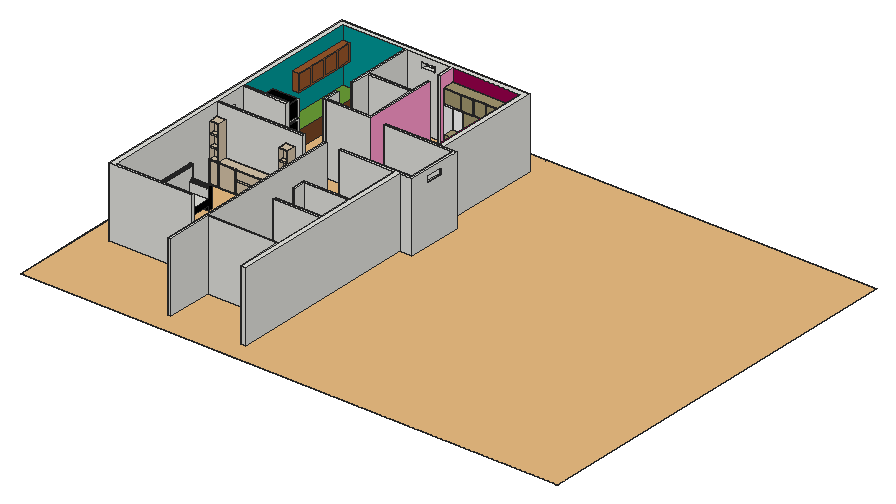
# SketchUp Ruby script. Lengths in millimetres.
U = 1.mm
M = Sketchup.active_model
def pt(a) = Geom::Point3d.new(a.map { |v| v * U })
def face(e, loops, mat)
  f = e.add_face(loops[0].map { |a| pt(a) })
  loops[1..].each { |l| e.add_face(l.map { |a| pt(a) }).erase! }
  f.material = f.back_material = mat if mat
  f
end
# faces: each face lists its corners as indices into pts; further lists are holes
def faces(e, pts, list, mat = nil) = list.each { |f| face(e, (f[0].is_a?(Array) ? f : [f]).map { |l| l.map { |i| pts[i] } }, mat) }
# xy, xz, yz: faces in a plane at the given z, y or x. An outline is a flat list of corners, or four numbers for a rectangle; further outlines are holes
def ring(l) = l.size == 4 ? [[l[0], l[1]], [l[2], l[1]], [l[2], l[3]], [l[0], l[3]]] : l.each_slice(2).to_a
def flat(e, list, mat, &to3) = list.each { |f| face(e, (f[0].is_a?(Array) ? f : [f]).map { |l| ring(l).map { |u, v| to3.(u, v) } }, mat) }
def xy(e, z, list, mat = nil) = flat(e, list, mat) { |x, y| [x, y, z] }
def xz(e, y, list, mat = nil) = flat(e, list, mat) { |x, z| [x, y, z] }
def yz(e, x, list, mat = nil) = flat(e, list, mat) { |y, z| [x, y, z] }
def lines(e, pts, list) = list.each { |a, b| e.add_line(pt(pts[a]), pt(pts[b])) }
# prism: a flat outline (further loops are holes) pulled along v
def prism(e, loops, v, mat = nil)
  f = face(e, loops, mat); d = Geom::Vector3d.new(v.map { |x| x * U })
  f.pushpull(f.normal.samedirection?(d) ? d.length : -d.length)
end
def box(e, o, s, mat = nil) = prism(e, [[o, [o[0] + s[0], o[1], o[2]], [o[0] + s[0], o[1] + s[1], o[2]], [o[0], o[1] + s[1], o[2]]]], [0, 0, s[2]], mat)
def at(x, y, z, deg = 0) = Geom::Transformation.translation(pt([x, y, z])) * Geom::Transformation.rotation(ORIGIN, Z_AXIS, deg.degrees)
def axes(o, x, y, z) = Geom::Transformation.new([*x, 0, *y, 0, *z, 0, *pt(o).to_a, 1])
def part(name) = M.definitions.add(name)
# library, detail: a bought-in or finely detailed component or shape, given as its bounding box
def library(name, o, s) = part(name).tap { |d| box(d.entities, o, s) }
def detail(e, o, s) = box(e.add_group.entities, o, s)
def put(e, d, t, mat = nil) = e.add_instance(d, t).tap { |i| i.material = mat if mat }
def group(e, t, mat = nil) = e.add_group.tap { |g| g.transformation = t; g.material = mat if mat }.entities
root = M.entities
M.materials.add("[Color H01]").color = [204, 255, 255]
M.materials.add("[Color H07]").color = [0, 153, 153]
M.materials.add("[Color L02]").color = [255, 153, 204]
M.materials.add("[Color L11]").color = [153, 0, 76]
M.materials.add("[Color M00]").color = [255, 255, 255]
M.materials.add("[Color M09]").color = [0, 0, 0]
M.materials.add("[Grass Dark Green]").color = [106, 157, 55]
M.materials.add("[Ornate Tile 02]").color = [201, 201, 201]
M.materials.add("[Tile Various Tan]").color = [214, 196, 169]
M.materials.add("[Wood Cherry Original]").color = [152, 86, 42]
M.materials.add("[Wood Lumber ButtJoined]").color = [164, 152, 112]
M.materials.add("[Wood Veneer 01]").color = [120, 70, 37]
c1 = library("DAY 6-A.dwg",[0,0,0],[23541.1,17455.5,0.1])
c2 = part("Component\#1")
xy(c2.entities,0,[[0,0,1144.4,1143]])
xy(c2.entities,1942.2,[[0,0,1144.4,40]])
xy(c2.entities,2054.6,[[0,0,1144.4,40]])
xy(c2.entities,3009.9,[[0,0,1144.4,1143]],"[Color M09]")
xz(c2.entities,0,[[[0,0,1144.4,1942.2],[23.7,24.4,1120.8,1917.8]],[[0,2054.6,1144.4,3009.9],[22.4,2077.6,1122.1,2986.9]]])
xz(c2.entities,0,[[23.7,24.4,1120.8,1917.8],[22.4,2077.6,1122.1,2986.9]],"[Color M09]")
xz(c2.entities,40,[[0,1942.2,1144.4,2054.6]],"[Color M09]")
xz(c2.entities,1143,[[0,0,1144.4,3009.9]],"[Color M09]")
yz(c2.entities,0,[[0,0,0,1942.2,40,1942.2,40,2054.6,0,2054.6,0,3009.9,1143,3009.9,1143,0]],"[Color M09]")
yz(c2.entities,1144.4,[[0,0,1143,0,1143,3009.9,0,3009.9,0,2054.6,40,2054.6,40,1942.2,0,1942.2]],"[Color M09]")
c3 = part("Single bed")
xy(c3.entities,0,[[0,0,1825,3282]])
xy(c3.entities,37.9,[[37.9,0,1787.1,38]],"[Wood Veneer 01]")
xy(c3.entities,85.7,[[0,85.7,53,3196.3],[1787,85.7,1825,3196.3]],"[Wood Veneer 01]")
xy(c3.entities,914.3,[[0,85.7,53,3196.3]])
xy(c3.entities,914.3,[[1787,85.7,1825,3196.3]],"[Wood Veneer 01]")
xy(c3.entities,962.1,[[37.9,0,1787.1,38]],"[Wood Veneer 01]")
xy(c3.entities,993.9,[[[122.3,122.3,1702.7,3153.7],[1037.3,2774.4,1637.3,3074.4],[237.3,2774.4,837.3,3074.4]]])
xy(c3.entities,993.9,[[146.1,3153.7,1678.9,3218.7]],"[Wood Veneer 01]")
xy(c3.entities,1000,[[0,0,1825,0,1825,3153.7,1702.7,3153.7,1702.7,122.3,122.3,122.3,122.3,3153.7,0,3153.7]],"[Wood Veneer 01]")
xy(c3.entities,1023.9,[[23.9,3153.7,146.1,3218.7],[1678.9,3153.7,1801.1,3218.7]],"[Wood Veneer 01]")
xy(c3.entities,1032.9,[[237.3,2774.4,837.3,3074.4],[1037.3,2774.4,1637.3,3074.4]])
xy(c3.entities,2018.1,[[23.9,3153.7,1801.1,3218.7]],"[Wood Veneer 01]")
xy(c3.entities,2042,[[0,3153.7,1825,3282]],"[Wood Veneer 01]")
xz(c3.entities,0,[[[0,0,1825,1000],[37.9,37.9,1787.1,962.1]]],"[Wood Veneer 01]")
xz(c3.entities,38,[[37.9,37.9,1787.1,962.1]],"[Wood Veneer 01]")
xz(c3.entities,85.7,[[0,85.7,53,914.3]])
xz(c3.entities,85.7,[[1787,85.7,1825,914.3]],"[Wood Veneer 01]")
xz(c3.entities,122.3,[[122.3,993.9,1702.7,1000]])
xz(c3.entities,2774.4,[[237.3,993.9,837.3,1032.9],[1037.3,993.9,1637.3,1032.9]])
xz(c3.entities,3074.4,[[237.3,993.9,837.3,1032.9],[1037.3,993.9,1637.3,1032.9]])
xz(c3.entities,3153.7,[[122.3,993.9,146.1,993.9,146.1,1023.9,23.9,1023.9,23.9,2018.1,1801.1,2018.1,1801.1,1023.9,1678.9,1023.9,1678.9,993.9,1702.7,993.9,1702.7,1000,1825,1000,1825,2042,0,2042,0,1000,122.3,1000]],"[Wood Veneer 01]")
xz(c3.entities,3196.3,[[0,85.7,53,914.3],[1787,85.7,1825,914.3]],"[Wood Veneer 01]")
xz(c3.entities,3218.7,[[146.1,993.9,1678.9,993.9,1678.9,1023.9,1801.1,1023.9,1801.1,2018.1,23.9,2018.1,23.9,1023.9,146.1,1023.9]])
xz(c3.entities,3282,[[0,0,1825,2042]],"[Wood Veneer 01]")
yz(c3.entities,0,[[[0,0,0,1000,3153.7,1000,3153.7,2042,3282,2042,3282,0],[85.7,85.7,3196.3,914.3]]],"[Wood Veneer 01]")
yz(c3.entities,23.9,[[3153.7,1023.9,3218.7,2018.1]],"[Wood Veneer 01]")
yz(c3.entities,37.9,[[0,37.9,38,962.1]],"[Wood Veneer 01]")
yz(c3.entities,53,[[85.7,85.7,3196.3,914.3]],"[Wood Veneer 01]")
yz(c3.entities,122.3,[[122.3,993.9,3153.7,1000]])
yz(c3.entities,146.1,[[3153.7,993.9,3218.7,1023.9]],"[Wood Veneer 01]")
yz(c3.entities,237.3,[[2774.4,993.9,3074.4,1032.9]])
yz(c3.entities,837.3,[[2774.4,993.9,3074.4,1032.9]])
yz(c3.entities,1037.3,[[2774.4,993.9,3074.4,1032.9]])
yz(c3.entities,1637.3,[[2774.4,993.9,3074.4,1032.9]])
yz(c3.entities,1678.9,[[3153.7,993.9,3218.7,1023.9]],"[Wood Veneer 01]")
yz(c3.entities,1702.7,[[122.3,993.9,3153.7,1000]])
yz(c3.entities,1787,[[85.7,85.7,3196.3,914.3]],"[Wood Veneer 01]")
yz(c3.entities,1787.1,[[0,37.9,38,962.1]],"[Wood Veneer 01]")
yz(c3.entities,1801.1,[[3153.7,1023.9,3218.7,2018.1]],"[Wood Veneer 01]")
yz(c3.entities,1825,[[[0,0,3282,0,3282,2042,3153.7,2042,3153.7,1000,0,1000],[85.7,85.7,3196.3,914.3]]],"[Wood Veneer 01]")
c4 = part("Component\#3")
xy(c4.entities,0,[[0,18,6874,2466]])
xy(c4.entities,99.3,[[99.3,0,6774.7,18]],"[Wood Veneer 01]")
xy(c4.entities,140.9,[[140.9,0,1757.8,18],[1840.9,0,5033.1,18],[5116.2,0,6733.1,18]],"[Wood Veneer 01]")
xy(c4.entities,1709.1,[[1840.9,0,5033.1,18]],"[Wood Veneer 01]")
xy(c4.entities,1792.2,[[1840.9,0,5033.1,18]],"[Wood Veneer 01]")
xy(c4.entities,3359.1,[[140.9,0,1757.8,18],[1840.9,0,5033.1,18],[5116.2,0,6733.1,18]],"[Wood Veneer 01]")
xy(c4.entities,3400.7,[[99.3,0,6774.7,18]],"[Wood Veneer 01]")
xy(c4.entities,3500,[[0,18,6874,2466]],"[Wood Veneer 01]")
xz(c4.entities,0,[[[99.3,99.3,6774.7,3400.7],[5116.2,140.9,6733.1,3359.1],[140.9,140.9,1757.8,3359.1],[1840.9,140.9,5033.1,1709.1],[1840.9,1792.2,5033.1,3359.1]]],"[Wood Veneer 01]")
xz(c4.entities,18,[[[0,0,6874,3500],[99.3,99.3,6774.7,3400.7]],[140.9,140.9,1757.8,3359.1],[1840.9,140.9,5033.1,1709.1],[5116.2,140.9,6733.1,3359.1],[1840.9,1792.2,5033.1,3359.1]],"[Wood Veneer 01]")
xz(c4.entities,2466,[[0,0,6874,3500]])
yz(c4.entities,0,[[18,0,2466,3500]],"[Wood Veneer 01]")
yz(c4.entities,99.3,[[0,99.3,18,3400.7]],"[Wood Veneer 01]")
yz(c4.entities,140.9,[[0,140.9,18,3359.1]],"[Wood Veneer 01]")
yz(c4.entities,1757.8,[[0,140.9,18,1750.7],[0,1750.7,18,3359.1]],"[Wood Veneer 01]")
yz(c4.entities,1840.9,[[0,140.9,18,1709.1],[0,1792.2,18,3359.1]],"[Wood Veneer 01]")
yz(c4.entities,5033.1,[[0,140.9,18,1709.1],[0,1792.2,18,3359.1]],"[Wood Veneer 01]")
yz(c4.entities,5116.2,[[0,140.9,18,1750.7],[0,1750.7,18,3359.1]],"[Wood Veneer 01]")
yz(c4.entities,6733.1,[[0,140.9,18,3359.1]],"[Wood Veneer 01]")
yz(c4.entities,6774.7,[[0,99.3,18,3400.7]],"[Wood Veneer 01]")
yz(c4.entities,6874,[[18,0,2466,3500]],"[Wood Veneer 01]")
c5 = part("High back sofa")
xy(c5.entities,0,[[0,0,0,1816,4458,1816,4458,1549,4457,1549,4457,0,4057,0,4057,1445,400,1445,400,0]],"[Color M09]")
xy(c5.entities,500,[[400,0,4057,1445]],"[Color M09]")
xy(c5.entities,1161,[[400,0,4057,1549]])
xy(c5.entities,2115,[[0,0,0.5,1549],[399.5,0,400,1549]])
xy(c5.entities,2150,[[4057,0,4057.5,1549],[4456.5,0,4457,1549]])
xz(c5.entities,0,[[4057,2131.5,4057,2138.2,4056.8,2132.6],[4057,2138.2,4057.5,2150,4057,2150]])
xz(c5.entities,0,[[0,0,400,0,400,500,4057,500,4057,0,4457,0,4457,2150,4456.5,2150,4457.2,2167.4,4445.9,2218.6,4421.7,2265.2,4386.3,2303.9,4342.1,2332.1,4292.1,2347.9,4257,2349.5,4239.6,2350.2,4188.4,2338.9,4141.8,2314.7,4103.1,2279.3,4074.9,2235.1,4059.1,2185.1,4057.5,2150,4057,2138.2,4057,1161,400,1161,400,2115,399.5,2115,392.7,2166.6,372.7,2214.7,341,2256,299.7,2287.7,251.6,2307.7,200,2314.5,148.4,2307.7,100.3,2287.7,59,2256,27.3,2214.7,7.3,2166.6,0.5,2115,0,2115]],"[Color M09]")
xz(c5.entities,1445,[[400,0,4057,500]],"[Color M09]")
xz(c5.entities,1549,[[4457,0,4458,0,4458,3496.2,4457,3496.2,4457,2168.5,4457.2,2167.4,4457,2161.8],[400,1161,4057,1161,4057,2150,4057.5,2150,4059.1,2185.1,4074.9,2235.1,4103.1,2279.3,4141.8,2314.7,4188.4,2338.9,4239.6,2350.2,4257,2349.5,4292.1,2347.9,4342.1,2332.1,4386.3,2303.9,4421.7,2265.2,4445.9,2218.6,4457,2168.5,4457,3496.2,0,3496.2,0,2115,0.5,2115,7.3,2166.6,27.3,2214.7,59,2256,100.3,2287.7,148.4,2307.7,200,2314.5,251.6,2307.7,299.7,2287.7,341,2256,372.7,2214.7,392.7,2166.6,399.5,2115,400,2115],[4456.5,2150,4457,2150,4457,2161.8]])
xz(c5.entities,1816,[[0,0,4458,3496.2]],"[Color M09]")
yz(c5.entities,0,[[0,0,0,2115,1549,2115,1549,3496.2,1548.5,3500,1553.1,3534.7,1566.5,3567,1587.7,3594.8,1615.5,3616,1647.8,3629.4,1682.5,3634,1717.2,3629.4,1749.5,3616,1777.3,3594.8,1798.5,3567,1811.9,3534.7,1816.5,3500,1816,3496.2,1816,0]],"[Color M09]")
yz(c5.entities,400,[[0,1161,1549,2115]])
yz(c5.entities,400,[[0,0,1445,500]],"[Color M09]")
yz(c5.entities,4057,[[0,1161,1549,2150]])
yz(c5.entities,4057,[[0,0,1445,500]],"[Color M09]")
yz(c5.entities,4457,[[0,0,1549,2150]],"[Color M09]")
yz(c5.entities,4458,[[1549,0,1816,0,1816,3496.2,1816.5,3500,1811.9,3534.7,1798.5,3567,1777.3,3594.8,1749.5,3616,1717.2,3629.4,1682.5,3634,1647.8,3629.4,1615.5,3616,1587.7,3594.8,1566.5,3567,1553.1,3534.7,1548.5,3500,1549,3496.2]],"[Color M09]")
p = [[0.5,0,2115],[7.3,0,2166.6],[7.3,1549,2166.6],[0.5,1549,2115],[392.7,0,2166.6],[399.5,0,2115],
  [399.5,1549,2115],[392.7,1549,2166.6],[4057.5,0,2150],[4059.1,0,2185.1],[4059.1,1549,2185.1],[4057.5,1549,2150],
  [4457.2,0,2167.4],[4456.5,0,2150],[4456.5,1549,2150],[4457,1549,2161.8],[4457.2,1549,2167.4],[27.3,0,2214.7],
  [27.3,1549,2214.7],[372.7,0,2214.7],[372.7,1549,2214.7],[4445.9,0,2218.6],[4457,1549,2168.5],[4445.9,1549,2218.6],
  [4074.9,0,2235.1],[4074.9,1549,2235.1],[59,0,2256],[59,1549,2256],[341,0,2256],[341,1549,2256],
  [4421.7,0,2265.2],[4421.7,1549,2265.2],[4103.1,0,2279.3],[4103.1,1549,2279.3],[100.3,0,2287.7],[100.3,1549,2287.7],
  [299.7,0,2287.7],[299.7,1549,2287.7],[4386.3,0,2303.9],[4386.3,1549,2303.9],[4141.8,0,2314.7],[4141.8,1549,2314.7],
  [148.4,0,2307.7],[148.4,1549,2307.7],[251.6,0,2307.7],[251.6,1549,2307.7],[4342.1,0,2332.1],[4342.1,1549,2332.1],
  [200,0,2314.5],[200,1549,2314.5],[4188.4,0,2338.9],[4188.4,1549,2338.9],[4292.1,0,2347.9],[4292.1,1549,2347.9],
  [4239.6,0,2350.2],[4239.6,1549,2350.2],[4257,0,2349.5],[4257,1549,2349.5],[4458,1549,3496.2],[4458,1548.5,3500],
  [4457,1548.5,3500],[0,1548.5,3500],[0,1549,3496.2],[4457,1549,3496.2],[4457,1816,3496.2],[0,1816,3496.2],
  [0,1816.5,3500],[4457,1816.5,3500],[4458,1816.5,3500],[4458,1816,3496.2],[4458,1553.1,3534.7],[4457,1553.1,3534.7],
  [0,1553.1,3534.7],[0,1811.9,3534.7],[4457,1811.9,3534.7],[4458,1811.9,3534.7],[4458,1566.5,3567],[4457,1566.5,3567],
  [0,1566.5,3567],[0,1798.5,3567],[4457,1798.5,3567],[4458,1798.5,3567],[4458,1587.7,3594.8],[4457,1587.7,3594.8],
  [0,1587.7,3594.8],[0,1777.3,3594.8],[4457,1777.3,3594.8],[4458,1777.3,3594.8],[4458,1615.5,3616],[4457,1615.5,3616],
  [0,1615.5,3616],[0,1749.5,3616],[4457,1749.5,3616],[4458,1749.5,3616],[4458,1647.8,3629.4],[4457,1647.8,3629.4],
  [0,1647.8,3629.4],[0,1717.2,3629.4],[4457,1717.2,3629.4],[4458,1717.2,3629.4],[4458,1682.5,3634],[4457,1682.5,3634],
  [0,1682.5,3634],[0,1549,3500],[4458,1816,3500],[4458,1549,3500],[0,1816,3500]]
faces(c5.entities,p,[[0,1,2,3],[4,5,6,7],[8,9,10,11],[12,13,14,15,16],[1,17,18,2],[19,4,7,20],[21,12,16,22,23],[9,24,25,10],
  [17,26,27,18],[28,19,20,29],[30,21,23,31],[24,32,33,25],[26,34,35,27],[36,28,29,37],[38,30,31,39],[32,40,41,33],
  [34,42,43,35],[44,36,37,45],[46,38,39,47],[42,48,49,43],[48,44,45,49],[40,50,51,41],[52,46,47,53],[50,54,55,51],
  [54,56,52,53,57,55],[58,59,60,61,62,63],[64,65,66,67,68,69],[59,70,71,72,61,60],[67,66,73,74,75,68],[70,76,77,78,72,71],[74,73,79,80,81,75],[76,82,83,84,78,77],
  [80,79,85,86,87,81],[82,88,89,90,84,83],[86,85,91,92,93,87],[88,94,95,96,90,89],[92,91,97,98,99,93],[94,100,101,102,96,95],[98,97,102,101,100,99]])
lines(c5.entities,p,[[62,103],[104,69],[58,105],[65,106]])
xy(root,0,[[5752.5,0,9144,914.4],[9144,0,10058.4,9330.7],[5752.5,914.4,5866.8,914.4,5866.8,2924.5,8915.4,2924.5,8915.4,914.4,9144,914.4,9144,9330.7,9699,9330.7,9699,11761.5,8915.4,11761.5,8915.4,11764.5,6613,11764.5,6613,11644.3,9582.5,11644.3,9582.5,9445,6484.9,9445,6484.9,9330.7,8915.4,9330.7,8915.4,6883.3,6895,6883.3,6895,6278.7,7009.3,6278.7,7009.3,6769,8915.4,6769,8915.4,5351.2,6895,5351.2,6895,5236.9,8915.4,5236.9,8915.4,2989.1,5866.8,2989.1,5866.8,9445,5752.5,9445],[5866.8,914.4,8915.4,2924.5],[0,3721,914.4,17373.6],
  [914.4,3721,4548.3,3721,4548.3,3835.3,1143,3835.3,1143,9330.7,4892.3,9330.7,4892.3,9445,1143,9445,1143,10735.8,3064,10735.8,3064,10850.1,1143,10850.1,1143,12376.4,1987.7,12376.4,1987.7,15654.3,3121.4,15654.3,3121.4,16230.6,3848.1,16230.6,3848.1,13280.6,3962.6,13280.6,3962.6,14054.7,3962.4,14054.7,3962.4,14164.8,3962.6,14164.8,3962.6,16230.6,5843.4,16230.6,5843.4,15559.9,5957.7,15559.9,5957.7,16230.6,8915.4,16230.6,8915.4,11764.5,9144,11764.5,9144,16459.2,914.4,16459.2],[9699,9330.7,10058.4,11761.5],[8915.4,11761.5,9144,11764.5],[9144,11761.5,9582.5,11764.5],[9699,11761.5,10058.4,11761.5,10058.4,17373.6,9144,17373.6,9144,11764.5,9699,11764.5],
  [9582.5,11761.5,9699,11764.5],[3962.4,14054.7,3962.6,14164.8],[5843.4,14054.7,5843.6,14164.8],[914.4,16459.2,9144,17373.6]])
xy(root,0,[[0,0,5752.5,3721]],"[Ornate Tile 02]")
xy(root,0,[[5866.8,2989.1,8915.4,2989.1,8915.4,5236.9,6895,5236.9,6895,5351.2,8915.4,5351.2,8915.4,6769,7009.3,6769,7009.3,6278.7,6895,6278.7,6895,6883.3,8915.4,6883.3,8915.4,9330.7,6484.9,9330.7,6484.9,9445,9582.5,9445,9582.5,11644.3,7124.1,11644.3,7124.1,10557.4,6616.1,10557.4,6616.1,11644.3,6613,11644.3,6613,11764.5,8915.4,11764.5,8915.4,15723.6,5957.7,15723.6,5957.7,15559.9,5843.4,15559.9,5843.4,16230.6,3962.6,16230.6,3962.6,14164.8,5843.4,14164.8,5843.4,14992.8,5957.7,14992.8,5957.7,11764.5,3962.6,11764.5,3962.6,11878.8,5843.4,11878.8,5843.4,14054.7,3962.6,14054.7,3962.6,13280.6,3848.1,13280.6,3848.1,15654.3,1987.7,15654.3,1987.7,12376.4,1143,12376.4,1143,10850.1,3064,10850.1,3064,10735.8,1143,10735.8,1143,9445,4892.3,9445,4892.3,9330.7,4562.1,9330.7,4562.1,8916.8,1143,8916.8,1143,3835.3,4548.3,3835.3,4548.3,3721,5752.5,3721,5752.5,9445,5866.8,9445]],"[Tile Various Tan]")
xy(root,9.4,[[5967,15723.6,6356.5,15730.6],[6416.5,15723.6,6806,15730.6],[6824.8,15723.6,7506,15730.6],[7524.8,15723.6,8206,15730.6],[8224.8,15723.6,8906,15730.6]],"[Color M00]")
xy(root,17.8,[[1160.8,8916.8,1526.2,8934.8],[1561.8,8916.8,2276.2,8934.8]],"[Tile Various Tan]")
xy(root,19.1,[[2313.1,8916.8,3393.9,8934.8]],"[Tile Various Tan]")
xy(root,20.3,[[3433.4,8916.8,4141.8,8934.8],[4183.4,8916.8,4541.8,8934.8]],"[Tile Various Tan]")
xy(root,27.4,[[3148.8,15654.3,3820.7,16280.3]],"[Wood Veneer 01]")
xy(root,300,[[2620.8,15881.8,2639.2,15884.2,2656.3,15891.3,2671,15902.6,2682.3,15917.3,2689.4,15934.4,2691.8,15952.8,2689.4,15971.2,2682.3,15988.3,2671,16003,2656.3,16014.3,2639.2,16021.4,2620.8,16023.8,2602.5,16021.4,2585.3,16014.3,2570.6,16003,2559.4,15988.3,2552.3,15971.2,2549.8,15952.8,2552.3,15934.4,2559.4,15917.3,2570.6,15902.6,2585.3,15891.3,2602.5,15884.2]])
xy(root,429.4,[[5967,15723.6,6356.5,15730.6],[6416.5,15723.6,6806,15730.6]],"[Color M00]")
xy(root,454.4,[[5967,15723.6,6806,15730.6]],"[Color M00]")
xy(root,475,[[[2293.1,15723.6,2968.9,16164.4],[2620.8,15881.8,2602.5,15884.2,2585.3,15891.3,2570.6,15902.6,2559.4,15917.3,2552.3,15934.4,2549.8,15952.8,2552.3,15971.2,2559.4,15988.3,2570.6,16003,2585.3,16014.3,2602.5,16021.4,2620.8,16023.8,2639.2,16021.4,2656.3,16014.3,2671,16003,2682.3,15988.3,2689.4,15971.2,2691.8,15952.8,2689.4,15934.4,2682.3,15917.3,2671,15902.6,2656.3,15891.3,2639.2,15884.2]]])
xy(root,530.9,[[2313.1,8916.8,3393.9,8934.8]],"[Tile Various Tan]")
xy(root,569.1,[[2313.1,8916.8,3393.9,8934.8]],"[Tile Various Tan]")
xy(root,663.5,[[5967,15730.6,6806,16168.6]],"[Wood Lumber ButtJoined]")
xy(root,672.6,[[3148.8,15654.3,3820.7,16280.3]])
xy(root,700,[[[1143,12376.4,1987.7,12376.4,1987.7,15654.3,3848.1,15654.3,3848.1,16230.6,1143,16230.6],[2267,15697.5,2995,16190.5]]],"[Grass Dark Green]")
xy(root,704,[[[2267,15697.5,2995,16190.5],[2293.1,15723.6,2968.9,16164.4]]])
xy(root,979.7,[[3433.4,8916.8,4141.8,8934.8],[4183.4,8916.8,4541.8,8934.8]],"[Tile Various Tan]")
xy(root,980.9,[[2313.1,8916.8,3393.9,8934.8]],"[Tile Various Tan]")
xy(root,982.2,[[1160.8,8916.8,1526.2,8934.8],[1561.8,8916.8,2276.2,8934.8]],"[Tile Various Tan]")
xy(root,1000,[[1143,8916.8,1543,8934.8],[1543,8916.8,4162.1,9330.7],[4162.1,8916.8,4562.1,8934.8]],"[Tile Various Tan]")
xy(root,1015.7,[[1158.7,8934.8,1527.3,9157.8],[4177.8,8934.8,4546.3,9157.8]],"[Tile Various Tan]")
xy(root,1484.3,[[1158.7,8934.8,1527.3,9157.8],[4177.8,8934.8,4546.3,9157.8]],"[Tile Various Tan]")
xy(root,1515.7,[[1158.7,8934.8,1527.3,9157.8],[4177.8,8934.8,4546.3,9157.8]],"[Tile Various Tan]")
xy(root,1718,[[1143,13430.6,1449,16230.6]])
xy(root,1741.7,[[1443,13454.3,1449,14106.9],[1443,14154.3,1449,14806.9],[1443,14854.3,1449,15506.9],[1443,15554.3,1449,16206.9]],"[Wood Cherry Original]")
xy(root,1840.6,[[5967,15723.6,6715.4,16168.6],[6715.4,15723.6,6806,16168.6],[6824.8,15723.6,7265.4,15730.6],[7265.4,15723.6,7506,15730.6],[7524.8,15723.6,7815.4,15730.6],
  [7815.4,15723.6,8206,15730.6],[8224.8,15723.6,8365.4,15730.6],[8365.4,15723.6,8906,15730.6]],"[Color M00]")
xy(root,1859.4,[[5967,15723.6,6706,15730.6],[6724.8,15723.6,6815.4,15730.6],[6815.4,15723.6,7256,15730.6],[7274.8,15723.6,7515.4,15730.6],[7515.4,15723.6,7806,15730.6],
  [7824.8,15723.6,8215.4,15730.6],[8215.4,15723.6,8356,15730.6],[8374.8,15723.6,8906,15730.6]],"[Color M00]")
xy(root,1984.3,[[1158.7,8934.8,1527.3,9157.8],[4177.8,8934.8,4546.3,9157.8]],"[Tile Various Tan]")
xy(root,2015.7,[[1158.7,8934.8,1527.3,9157.8],[4177.8,8934.8,4546.3,9157.8]],"[Tile Various Tan]")
xy(root,2332.1,[[914.4,9911,1143,10360]])
xy(root,2444.3,[[1443,13454.3,1449,14106.9],[1443,14154.3,1449,14806.9],[1443,14854.3,1449,15506.9],[1443,15554.3,1449,16206.9]],"[Wood Cherry Original]")
xy(root,2466.9,[[9582.5,10139.4,9699,10982.4]])
xy(root,2468,[[1143,13430.6,1449,16230.6]],"[Wood Cherry Original]")
xy(root,2484.3,[[1158.7,8934.8,1527.3,9157.8],[4177.8,8934.8,4546.3,9157.8]],"[Tile Various Tan]")
xy(root,2490.6,[[5967,15723.6,6706,15730.6],[6724.8,15723.6,7256,15730.6],[7274.8,15723.6,7806,15730.6],[7824.8,15723.6,8356,15730.6],[8374.8,15723.6,8906,15730.6]],"[Color M00]")
xy(root,2500,[[1143,8934.8,1543,9330.7],[4162.1,8934.8,4562.1,9330.7]],"[Tile Various Tan]")
xy(root,2500,[[5957.7,15723.6,8915.4,16230.6]],"[Wood Lumber ButtJoined]")
xy(root,2571.4,[[4607.3,16230.6,5189.3,16459.2]])
xy(root,2576.1,[[914.4,9911,1143,10360]])
xy(root,2784.9,[[9582.5,10139.4,9699,10982.4]])
xy(root,2828.4,[[4607.3,16230.6,5189.3,16459.2]])
xy(root,3048,[[5752.5,914.4,5866.8,914.4,5866.8,2924.5,8915.4,2924.5,8915.4,914.4,9144,914.4,9144,9330.7,9699,9330.7,9699,11761.5,8915.4,11761.5,8915.4,11764.5,6613,11764.5,6613,11644.3,9582.5,11644.3,9582.5,9445,6484.9,9445,6484.9,9330.7,8915.4,9330.7,8915.4,6883.3,6895,6883.3,6895,6278.7,7009.3,6278.7,7009.3,6769,8915.4,6769,8915.4,5351.2,6895,5351.2,6895,5236.9,8915.4,5236.9,8915.4,2989.1,5866.8,2989.1,5866.8,9445,5752.5,9445],[914.4,3721,4548.3,3721,4548.3,3835.3,1143,3835.3,1143,9330.7,4892.3,9330.7,4892.3,9445,1143,9445,1143,10735.8,3064,10735.8,3064,10850.1,1143,10850.1,1143,16230.6,3848.1,16230.6,3848.1,13280.6,3962.6,13280.6,3962.6,14054.7,3962.4,14054.7,3962.4,14164.8,3962.6,14164.8,3962.6,16230.6,5843.4,16230.6,5843.4,15559.9,5957.7,15559.9,5957.7,16230.6,8915.4,16230.6,8915.4,11764.5,9144,11764.5,9144,16459.2,914.4,16459.2],[3848.1,11764.5,3962.4,12495.9],[3962.6,11764.5,5957.7,11764.5,5957.7,14992.8,5843.4,14992.8,5843.4,14164.8,5843.6,14164.8,5843.6,14054.7,5843.4,14054.7,5843.4,11878.8,3962.6,11878.8],[3962.6,14054.7,5843.4,14164.8]])
xz(root,914.4,[[5752.5,0,5866.8,3048],[8915.4,0,9144,3048]])
xz(root,2924.5,[[5866.8,0,8915.4,3048]])
xz(root,2989.1,[[5866.8,0,8915.4,3048]])
xz(root,3721,[[914.4,0,4548.3,3048]])
xz(root,3835.3,[[1143,0,4548.3,3048]])
xz(root,5236.9,[[6895,0,8915.4,3048]])
xz(root,5351.2,[[6895,0,8915.4,3048]])
xz(root,6278.7,[[6895,0,7009.3,3048]])
xz(root,6769,[[7009.3,0,8915.4,3048]])
xz(root,6883.3,[[6895,0,7009.3,3048],[7009.3,0,8915.4,3048]])
xz(root,8916.8,[[[1143,0,4562.1,1000],[1561.8,17.8,2276.2,982.2],[3433.4,20.3,4141.8,979.7],[2313.1,19.1,3393.9,530.9],[2313.1,569.1,3393.9,980.9],[1160.8,17.8,1526.2,982.2],[4183.4,20.3,4541.8,979.7]]],"[Tile Various Tan]")
xz(root,8934.8,[[1160.8,17.8,1526.2,982.2],[1561.8,17.8,2276.2,982.2],[2313.1,19.1,3393.9,530.9],[3433.4,20.3,4141.8,979.7],[4183.4,20.3,4541.8,979.7],
  [2313.1,569.1,3393.9,980.9],[[1143,1000,1543,2500],[1158.7,2015.7,1527.3,2484.3],[1158.7,1515.7,1527.3,1984.3],[1158.7,1015.7,1527.3,1484.3]],[[4162.1,1000,4562.1,2500],[4177.8,2015.7,4546.3,2484.3],[4177.8,1515.7,4546.3,1984.3],[4177.8,1015.7,4546.3,1484.3]]],"[Tile Various Tan]")
xz(root,9157.8,[[1158.7,1015.7,1527.3,1484.3],[4177.8,1015.7,4546.3,1484.3],[1158.7,1515.7,1527.3,1984.3],[4177.8,1515.7,4546.3,1984.3],[1158.7,2015.7,1527.3,2484.3],
  [4177.8,2015.7,4546.3,2484.3]],"[Tile Various Tan]")
xz(root,9330.7,[[4562.1,0,4892.3,0,4892.3,3048,1143,3048,1143,2500,1543,2500,1543,1000,4162.1,1000,4162.1,2500,4562.1,2500],[6484.9,0,8915.4,3048],[9144,0,9699,3048]])
xz(root,9330.7,[[1143,0,4562.1,0,4562.1,2500,4162.1,2500,4162.1,1000,1543,1000,1543,2500,1143,2500]],"[Tile Various Tan]")
xz(root,9445,[[1143,0,4892.3,3048],[5752.5,0,5866.8,3048],[6484.9,0,9582.5,3048]])
xz(root,9911,[[914.4,2332.1,1143,2576.1]])
xz(root,10139.4,[[9582.5,2466.9,9699,2784.9]])
xz(root,10360,[[914.4,2332.1,1143,2576.1]])
xz(root,10735.8,[[1143,0,3064,3048]])
xz(root,10850.1,[[1143,0,3064,3048]],"[Color H07]")
xz(root,10982.4,[[9582.5,2466.9,9699,2784.9]])
xz(root,11644.3,[[6613,0,6616.1,3048],[6616.1,0,9582.5,3048]])
xz(root,11761.5,[[8915.4,0,9144,3048],[9144,0,9699,3048]])
xz(root,11764.5,[[3848.1,0,3962.4,3048],[3962.6,0,5957.7,3048],[8915.4,0,9144,3048]])
xz(root,11764.5,[[6613,0,8915.4,3048]],"[Color L11]")
xz(root,11878.8,[[3962.6,0,5843.4,3048]])
xz(root,12376.4,[[1143,0,1987.7,700]])
xz(root,12495.9,[[3848.1,0,3962.4,3048]])
xz(root,13280.6,[[3848.1,0,3962.6,3048]])
xz(root,13430.6,[[1143,1718,1449,2468]],"[Wood Cherry Original]")
xz(root,13454.3,[[1443,1741.7,1449,2444.3]],"[Wood Cherry Original]")
xz(root,14054.7,[[3962.4,0,3962.6,3048],[3962.6,0,5843.4,3048],[5843.4,0,5843.6,3048]])
xz(root,14106.9,[[1443,1741.7,1449,2444.3]],"[Wood Cherry Original]")
xz(root,14154.3,[[1443,1741.7,1449,2444.3]],"[Wood Cherry Original]")
xz(root,14164.8,[[3962.4,0,3962.6,3048],[3962.6,0,5843.4,3048],[5843.4,0,5843.6,3048]])
xz(root,14806.9,[[1443,1741.7,1449,2444.3]],"[Wood Cherry Original]")
xz(root,14854.3,[[1443,1741.7,1449,2444.3]],"[Wood Cherry Original]")
xz(root,14992.8,[[5843.4,0,5957.7,3048]])
xz(root,15506.9,[[1443,1741.7,1449,2444.3]],"[Wood Cherry Original]")
xz(root,15554.3,[[1443,1741.7,1449,2444.3]],"[Wood Cherry Original]")
xz(root,15559.9,[[5843.4,0,5957.7,3048]])
xz(root,15654.3,[[[1987.7,0,3848.1,700],[3148.8,27.4,3820.7,672.6]]],"[Wood Veneer 01]")
xz(root,15697.5,[[2267,700,2995,704]])
xz(root,15723.6,[[2293.1,475,2968.9,704]])
xz(root,15723.6,[[[5957.7,0,8915.4,2500],[5967,9.4,6806,1840.6],[8224.8,9.4,8906,1840.6],[6824.8,9.4,7506,1840.6],[7524.8,9.4,8206,1840.6],[5967,1859.4,6706,2490.6],[6724.8,1859.4,7256,2490.6],[7274.8,1859.4,7806,2490.6],[8374.8,1859.4,8906,2490.6],[7824.8,1859.4,8356,2490.6]],[6356.5,9.4,6416.5,9.4,6416.5,429.4,6806,429.4,6806,454.4,5967,454.4,5967,429.4,6356.5,429.4]],"[Color M00]")
xz(root,15730.6,[[5967,9.4,6356.5,429.4],[6416.5,9.4,6806,429.4],[6824.8,9.4,7506,1840.6],[7524.8,9.4,8206,1840.6],[8224.8,9.4,8906,1840.6],
  [5967,454.4,6806,663.5],[5967,1859.4,6706,2490.6],[6724.8,1859.4,7256,2490.6],[7274.8,1859.4,7806,2490.6],[7824.8,1859.4,8356,2490.6],
  [8374.8,1859.4,8906,2490.6]],"[Wood Lumber ButtJoined]")
xz(root,16164.4,[[2293.1,475,2968.9,704]])
xz(root,16190.5,[[2267,700,2995,704]])
xz(root,16206.9,[[1443,1741.7,1449,2444.3]],"[Wood Cherry Original]")
xz(root,16230.6,[[3121.4,0,3848.1,700],[[3962.6,0,5843.4,3048],[4607.3,2571.4,5189.3,2828.4]]])
xz(root,16230.6,[[1143,700,3848.1,700,3848.1,3048,1143,3048,1143,2468,1449,2468,1449,1718,1143,1718]],"[Color H07]")
xz(root,16230.6,[[5957.7,2500,8915.4,3048]],"[Color L11]")
xz(root,16230.6,[[5957.7,0,8915.4,2500]],"[Color M00]")
xz(root,16280.3,[[3148.8,27.4,3820.7,672.6]])
xz(root,16459.2,[[[914.4,0,9144,3048],[4607.3,2571.4,5189.3,2828.4]]])
yz(root,914.4,[[[3721,0,16459.2,3048],[9911,2332.1,10360,2576.1]]])
yz(root,1143,[[3835.3,0,8916.8,0,8916.8,1000,8934.8,1000,8934.8,2500,9330.7,2500,9330.7,3048,3835.3,3048],[[9445,0,10735.8,3048],[9911,2332.1,10360,2576.1]]])
yz(root,1143,[[10850.1,0,12376.4,0,12376.4,700,16230.6,700,16230.6,1718,13430.6,1718,13430.6,2468,16230.6,2468,16230.6,3048,10850.1,3048]],"[Color H07]")
yz(root,1143,[[8916.8,0,9330.7,0,9330.7,2500,8934.8,2500,8934.8,1000,8916.8,1000]],"[Tile Various Tan]")
yz(root,1158.7,[[8934.8,1015.7,9157.8,1484.3],[8934.8,1515.7,9157.8,1984.3],[8934.8,2015.7,9157.8,2484.3]],"[Tile Various Tan]")
yz(root,1160.8,[[8916.8,17.8,8934.8,982.2]],"[Tile Various Tan]")
yz(root,1443,[[13454.3,1741.7,14106.9,2444.3],[14154.3,1741.7,14806.9,2444.3],[14854.3,1741.7,15506.9,2444.3],[15554.3,1741.7,16206.9,2444.3]],"[Wood Cherry Original]")
yz(root,1449,[[[13430.6,1718,16230.6,2468],[14854.3,1741.7,15506.9,2444.3],[13454.3,1741.7,14106.9,2444.3],[15554.3,1741.7,16206.9,2444.3],[14154.3,1741.7,14806.9,2444.3]]],"[Wood Cherry Original]")
yz(root,1526.2,[[8916.8,17.8,8934.8,982.2]],"[Tile Various Tan]")
yz(root,1527.3,[[8934.8,1015.7,9157.8,1484.3],[8934.8,1515.7,9157.8,1984.3],[8934.8,2015.7,9157.8,2484.3]],"[Tile Various Tan]")
yz(root,1543,[[8934.8,1000,9330.7,2500]],"[Tile Various Tan]")
yz(root,1561.8,[[8916.8,17.8,8934.8,982.2]],"[Tile Various Tan]")
yz(root,1987.7,[[12376.4,0,15654.3,700]],"[Wood Veneer 01]")
yz(root,2267,[[15697.5,700,16190.5,704]])
yz(root,2276.2,[[8916.8,17.8,8934.8,550],[8916.8,550,8934.8,982.2]],"[Tile Various Tan]")
yz(root,2293.1,[[15723.6,475,16164.4,704]])
yz(root,2313.1,[[8916.8,19.1,8934.8,530.9],[8916.8,569.1,8934.8,980.9]],"[Tile Various Tan]")
yz(root,2968.9,[[15723.6,475,16164.4,704]])
yz(root,2995,[[15697.5,700,16190.5,704]])
yz(root,3064,[[10735.8,0,10850.1,3048]])
yz(root,3148.8,[[15654.3,27.4,16280.3,672.6]],"[Wood Veneer 01]")
yz(root,3393.9,[[8916.8,19.1,8934.8,530.9],[8916.8,569.1,8934.8,980.9]],"[Tile Various Tan]")
yz(root,3433.4,[[8916.8,20.3,8934.8,550],[8916.8,550,8934.8,979.7]],"[Tile Various Tan]")
yz(root,3820.7,[[15654.3,27.4,16280.3,672.6]],"[Wood Veneer 01]")
yz(root,3848.1,[[15654.3,0,16230.6,700]])
yz(root,3848.1,[[11764.5,0,12495.9,3048],[13280.6,0,13280.6,3048,16230.6,3048,16230.6,700,15654.3,700,15654.3,0]],"[Color H01]")
yz(root,3962.4,[[11764.5,0,12495.9,3048],[14054.7,0,14164.8,3048]])
yz(root,3962.6,[[11764.5,0,11878.8,3048],[13280.6,0,14054.7,3048],[14054.7,0,14164.8,3048],[14164.8,0,16230.6,3048]])
yz(root,4141.8,[[8916.8,20.3,8934.8,979.7]],"[Tile Various Tan]")
yz(root,4162.1,[[8934.8,1000,9330.7,2500]],"[Tile Various Tan]")
yz(root,4177.8,[[8934.8,1015.7,9157.8,1484.3],[8934.8,1515.7,9157.8,1984.3],[8934.8,2015.7,9157.8,2484.3]],"[Tile Various Tan]")
yz(root,4183.4,[[8916.8,20.3,8934.8,979.7]],"[Tile Various Tan]")
yz(root,4541.8,[[8916.8,20.3,8934.8,979.7]],"[Tile Various Tan]")
yz(root,4546.3,[[8934.8,1015.7,9157.8,1484.3],[8934.8,1515.7,9157.8,1984.3],[8934.8,2015.7,9157.8,2484.3]],"[Tile Various Tan]")
yz(root,4548.3,[[3721,0,3835.3,3048]])
yz(root,4562.1,[[8916.8,0,9330.7,0,9330.7,2500,8934.8,2500,8934.8,1000,8916.8,1000]],"[Tile Various Tan]")
yz(root,4607.3,[[16230.6,2571.4,16459.2,2828.4]])
yz(root,4892.3,[[9330.7,0,9445,3048]])
yz(root,5189.3,[[16230.6,2571.4,16459.2,2828.4]])
yz(root,5752.5,[[914.4,0,9445,3048]])
yz(root,5843.4,[[11878.8,0,14054.7,3048],[14054.7,0,14164.8,3048],[14164.8,0,14992.8,3048],[15559.9,0,16230.6,3048]])
yz(root,5843.6,[[14054.7,0,14164.8,3048]])
yz(root,5866.8,[[914.4,0,2924.5,3048],[2989.1,0,9445,3048]])
yz(root,5957.7,[[11764.5,0,14992.8,3048],[15559.9,0,15723.6,0,15723.6,2500,16230.6,2500,16230.6,3048,15559.9,3048]],"[Color L02]")
yz(root,5957.7,[[15723.6,0,16230.6,2500]],"[Color M00]")
yz(root,5967,[[15723.6,9.4,15730.6,429.4],[15723.6,454.4,15730.6,454.4,15730.6,663.5,16168.6,663.5,16168.6,1840.6,15723.6,1840.6],[15723.6,1859.4,15730.6,2490.6]],"[Color M00]")
yz(root,6356.5,[[15723.6,9.4,15730.6,429.4]],"[Color M00]")
yz(root,6416.5,[[15723.6,9.4,15730.6,429.4]],"[Color M00]")
yz(root,6484.9,[[9330.7,0,9445,3048]])
yz(root,6613,[[11644.3,0,11764.5,3048]])
yz(root,6706,[[15723.6,1859.4,15730.6,2490.6]],"[Color M00]")
yz(root,6724.8,[[15723.6,1859.4,15730.6,2490.6]],"[Color M00]")
yz(root,6806,[[15723.6,9.4,15730.6,429.4],[15723.6,454.4,15723.6,1840.6,16168.6,1840.6,16168.6,663.5,15730.6,663.5,15730.6,454.4]],"[Color M00]")
yz(root,6824.8,[[15723.6,9.4,15730.6,1840.6]],"[Color M00]")
yz(root,6895,[[5236.9,0,5351.2,3048],[6278.7,0,6883.3,3048]])
yz(root,7009.3,[[6278.7,0,6769,3048]])
yz(root,7256,[[15723.6,1859.4,15730.6,2490.6]],"[Color M00]")
yz(root,7274.8,[[15723.6,1859.4,15730.6,2490.6]],"[Color M00]")
yz(root,7506,[[15723.6,9.4,15730.6,1840.6]],"[Color M00]")
yz(root,7524.8,[[15723.6,9.4,15730.6,1840.6]],"[Color M00]")
yz(root,7806,[[15723.6,1859.4,15730.6,2490.6]],"[Color M00]")
yz(root,7824.8,[[15723.6,1859.4,15730.6,2490.6]],"[Color M00]")
yz(root,8206,[[15723.6,9.4,15730.6,1840.6]],"[Color M00]")
yz(root,8224.8,[[15723.6,9.4,15730.6,1840.6]],"[Color M00]")
yz(root,8356,[[15723.6,1859.4,15730.6,2490.6]],"[Color M00]")
yz(root,8374.8,[[15723.6,1859.4,15730.6,2490.6]],"[Color M00]")
yz(root,8906,[[15723.6,9.4,15730.6,1840.6],[15723.6,1859.4,15730.6,2490.6]],"[Color M00]")
yz(root,8915.4,[[914.4,0,2924.5,3048],[2989.1,0,5236.9,3048],[5351.2,0,6769,3048],[6883.3,0,9330.7,3048],[11761.5,0,11764.5,3048]])
yz(root,8915.4,[[11764.5,0,11764.5,3048,16230.6,3048,16230.6,2500,15723.6,2500,15723.6,0]],"[Color L11]")
yz(root,8915.4,[[15723.6,0,16230.6,2500]],"[Tile Various Tan]")
yz(root,9144,[[914.4,0,9330.7,3048],[11764.5,0,16459.2,3048]])
yz(root,9582.5,[[[9445,0,11644.3,3048],[10139.4,2466.9,10982.4,2784.9]]])
yz(root,9699,[[[9330.7,0,11761.5,3048],[10139.4,2466.9,10982.4,2784.9]]])
p = [[2602.5,15884.2,475],[2620.8,15881.8,475],[2620.8,15881.8,300],[2602.5,15884.2,300],[2639.2,15884.2,475],[2639.2,15884.2,300],
  [2585.3,15891.3,475],[2585.3,15891.3,300],[2656.3,15891.3,475],[2656.3,15891.3,300],[2570.6,15902.6,475],[2570.6,15902.6,300],
  [2671,15902.6,475],[2671,15902.6,300],[2559.4,15917.3,475],[2559.4,15917.3,300],[2682.3,15917.3,475],[2682.3,15917.3,300],
  [2552.3,15934.4,475],[2552.3,15934.4,300],[2689.4,15934.4,475],[2689.4,15934.4,300],[2549.8,15952.8,475],[2549.8,15952.8,300],
  [2691.8,15952.8,475],[2691.8,15952.8,300],[2552.3,15971.2,475],[2552.3,15971.2,300],[2689.4,15971.2,475],[2689.4,15971.2,300],
  [2559.4,15988.3,475],[2559.4,15988.3,300],[2682.3,15988.3,475],[2682.3,15988.3,300],[2570.6,16003,475],[2570.6,16003,300],
  [2671,16003,475],[2671,16003,300],[2585.3,16014.3,475],[2585.3,16014.3,300],[2656.3,16014.3,475],[2656.3,16014.3,300],
  [2602.5,16021.4,475],[2602.5,16021.4,300],[2639.2,16021.4,475],[2639.2,16021.4,300],[2620.8,16023.8,475],[2620.8,16023.8,300],
  [6867,10557.4,0],[6867,11644.3,0],[5967,15730.8,659.3],[6806,15723.6,663.5]]
faces(root,p,[[0,1,2,3],[1,4,5,2],[6,0,3,7],[4,8,9,5],[10,6,7,11],[8,12,13,9],[14,10,11,15],[12,16,17,13],
  [18,14,15,19],[16,20,21,17],[22,18,19,23],[20,24,25,21],[26,22,23,27],[24,28,29,25],[30,26,27,31],[28,32,33,29],
  [34,30,31,35],[32,36,37,33],[38,34,35,39],[36,40,41,37],[42,38,39,43],[40,44,45,41],[46,42,43,47],[44,46,47,45]])
lines(root,p,[[48,49],[50,51]])
put(root,c1,at(0,0,0))
put(root,c2,axes([2335,11182.3,38.1],[0,1,0],[-1,0,0],[0,0,0.7469]))
put(root,c3,axes([6738.2,15092.2,-51.9],[0,-0.8624,0],[0.6272,0,0],[0,0,0.6052]))
put(root,c4,axes([1697.1,9445,0],[0,0.18778,0],[-0.2868,0,0],[0,0,0.10455]))
put(root,c3,axes([6856.9,4740.3,0],[0,-0.8624,0],[0.6272,0,0],[0,0,0.6052]))
put(root,c5,axes([2295.5,5426.1,0],[0,0.49577,0],[-0.546,0,0],[0,0,0.40252]))
put(root,c5,axes([4186.2,4935,0],[-0.49577,0,0],[0,-0.546,0],[0,0,0.40252]))
